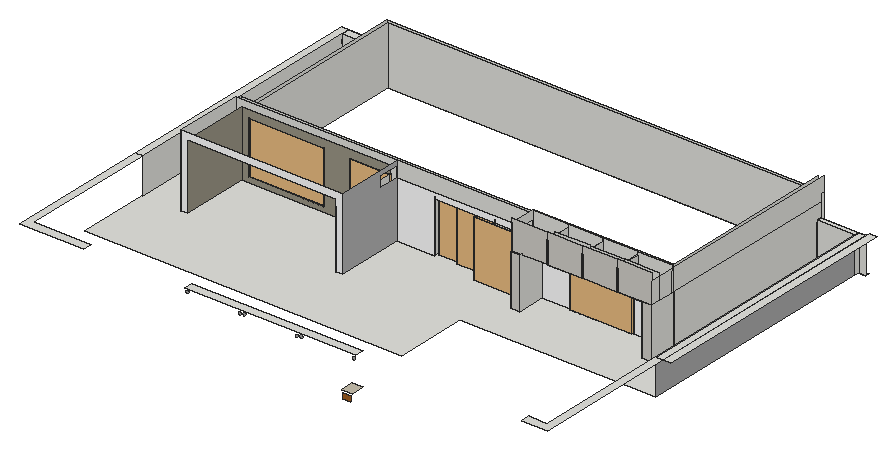
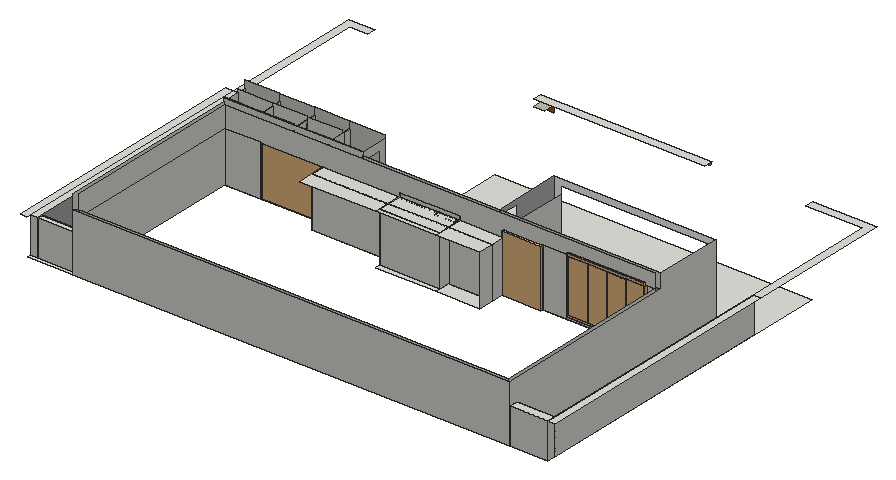
# SketchUp Ruby script. Lengths in inches.
U = 1.inch
M = Sketchup.active_model
def pt(a) = Geom::Point3d.new(a.map { |v| v * U })
def face(e, loops, mat)
  f = e.add_face(loops[0].map { |a| pt(a) })
  loops[1..].each { |l| e.add_face(l.map { |a| pt(a) }).erase! }
  f.material = f.back_material = mat if mat
  f
end
# faces: each face lists its corners as indices into pts; further lists are holes
def faces(e, pts, list, mat = nil) = list.each { |f| face(e, (f[0].is_a?(Array) ? f : [f]).map { |l| l.map { |i| pts[i] } }, mat) }
# xy, xz, yz: faces in a plane at the given z, y or x. An outline is a flat list of corners, or four numbers for a rectangle; further outlines are holes
def ring(l) = l.size == 4 ? [[l[0], l[1]], [l[2], l[1]], [l[2], l[3]], [l[0], l[3]]] : l.each_slice(2).to_a
def flat(e, list, mat, &to3) = list.each { |f| face(e, (f[0].is_a?(Array) ? f : [f]).map { |l| ring(l).map { |u, v| to3.(u, v) } }, mat) }
def xy(e, z, list, mat = nil) = flat(e, list, mat) { |x, y| [x, y, z] }
def xz(e, y, list, mat = nil) = flat(e, list, mat) { |x, z| [x, y, z] }
def yz(e, x, list, mat = nil) = flat(e, list, mat) { |y, z| [x, y, z] }
def lines(e, pts, list) = list.each { |a, b| e.add_line(pt(pts[a]), pt(pts[b])) }
# prism: a flat outline (further loops are holes) pulled along v
def prism(e, loops, v, mat = nil)
  f = face(e, loops, mat); d = Geom::Vector3d.new(v.map { |x| x * U })
  f.pushpull(f.normal.samedirection?(d) ? d.length : -d.length)
end
def box(e, o, s, mat = nil) = prism(e, [[o, [o[0] + s[0], o[1], o[2]], [o[0] + s[0], o[1] + s[1], o[2]], [o[0], o[1] + s[1], o[2]]]], [0, 0, s[2]], mat)
def at(x, y, z, deg = 0) = Geom::Transformation.translation(pt([x, y, z])) * Geom::Transformation.rotation(ORIGIN, Z_AXIS, deg.degrees)
def axes(o, x, y, z) = Geom::Transformation.new([*x, 0, *y, 0, *z, 0, *pt(o).to_a, 1])
def part(name) = M.definitions.add(name)
# library, detail: a bought-in or finely detailed component or shape, given as its bounding box
def library(name, o, s) = part(name).tap { |d| box(d.entities, o, s) }
def detail(e, o, s) = box(e.add_group.entities, o, s)
def put(e, d, t, mat = nil) = e.add_instance(d, t).tap { |i| i.material = mat if mat }
def group(e, t, mat = nil) = e.add_group.tap { |g| g.transformation = t; g.material = mat if mat }.entities
root = M.entities
M.materials.add("Material~3").color = [123, 113, 102]
M.materials.add("[0128_White]").color = [255, 255, 255]
M.materials.add("[0129_WhiteSmoke]").color = [178, 178, 178]
M.materials.add("[0132_LightGray]").color = [169, 169, 169]
M.materials.add("[Concrete Tile]").color = [155, 150, 134]
M.materials.add("[Terrazzo Tile Light]").color = [209, 207, 200]
M.materials.add("[Tile Canvas]").color = [199, 192, 173]
M.materials.add("[Wood Square Tile 02]").color = [160, 95, 34]
c1 = library("3DGeom~4_Defintion",[362.52,-15.59,12.6],[288.85,70.11,1000])
c2 = library("3 door",[0,0,0],[74.8,3.9375,43.31])
c3 = library("door (1)",[38.93,25.48,0],[40,9.94,82.68])
c4 = library("JALI+PATTERN-03",[8.875,53.125,6.4375],[84,1,53.5])
xy(root,5.1875,[[[288.55,611.53,816.46,611.53,816.46,732.28,1144.18,732.28,1144.18,1146.63,1080.92,1146.63,1080.92,851.0625,911.51,851.0625,911.51,845.35,864.05,845.35,864.05,798.41,848.72,798.41,848.72,845.35,784.44,845.35,784.44,874.25,684.16,874.25,684.16,845.35,621.47,845.35,621.47,732.28,610.53,732.28,610.53,851.0625,545.16,851.0625,545.16,845.35,363.11,845.35,363.11,732.28,352.17,732.28,352.17,1146.63,288.55,1146.63],[1065.59,801.78,1080.92,845.35]],[352.17,732.28,352.17,1160.85,1156.17,1160.85,1156.17,1155.13,357.89,1155.13,357.89,851.0625,545.16,851.0625,545.16,845.35,363.11,845.35,363.11,732.28],[610.53,732.28,610.53,846.1,684.16,846.1,684.16,845.35,621.47,845.35,621.47,732.28],[848.72,798.41,848.72,845.35,784.44,845.35,784.44,846.1,911.51,846.1,911.51,845.35,864.05,845.35,864.05,798.41],[1065.59,801.78,1080.92,845.35],
  [610.53,846.1,684.16,874.25],[784.44,846.1,911.51,874.25],[1075.21,851.0625,1080.92,1155.13],[610.53,874.25,684.16,900.375],[684.16,874.25,784.44,892.35],
  [684.16,892.35,784.44,900.375],[288.55,1146.63,352.17,1160.85],[1080.92,1146.63,1144.18,1155.13]])
xy(root,13.84,[[374.83,845.35,499.71,851.0625]])
xy(root,32.74,[[842.6875,453.42,861.125,475.99]],"[Tile Canvas]")
xy(root,65.1875,[[276.92,491.47,382.82,491.47,382.82,505.1,288.55,505.1,288.55,732.28,276.92,732.28],[551.82,491.47,836.67,505.1],[1113.48,491.47,1156.17,491.47,1156.17,732.28,1144.18,732.28,1144.18,505.1,1113.48,505.1],[276.92,732.28,288.55,1160.85],[1144.18,732.28,1156.17,1155.13],
  [1156.87,732.28,1168.49,1160.85],[288.55,1146.63,352.17,1160.85],[1080.92,1146.63,1144.18,1155.13]])
xy(root,89.42,[[848.72,798.41,864.05,801.78],[864.05,801.78,906.77,814.22],[907.71,801.78,911.51,817.6],[911.51,801.78,964.82,817.6],[965.89,801.78,1016.125,817.6],
  [1016.125,801.78,1022.875,817.6],[1024.1875,801.78,1065.59,817.6],[1065.59,801.78,1080.92,817.6],[864.05,814.22,906.77,844.47],[907.71,817.6,911.51,844.47],
  [911.51,817.6,964.82,844.47],[965.89,817.6,1016.125,844.47],[1016.125,817.6,1022.875,844.47],[1024.1875,817.6,1065.59,844.47],[1065.59,817.6,1080.92,844.47],
  [848.72,844.47,864.05,845.35],[864.05,844.47,911.51,845.35],[911.51,844.47,1016.125,845.35],[1016.125,844.47,1065.59,845.35],[1065.59,844.47,1080.92,845.35],
  [684.16,845.35,784.44,846.1],[784.44,845.35,848.72,846.1],[848.72,845.35,911.51,846.1],[911.51,845.35,1016.125,846.1],[1016.125,845.35,1080.92,846.1],
  [610.53,846.1,684.16,851.0625],[784.44,846.1,911.51,851.0625],[911.51,846.1,1016.125,851.0625],[1016.125,846.1,1080.92,851.0625],[610.53,851.0625,684.16,874.25],
  [684.16,851.0625,784.44,874.25],[784.44,851.0625,911.51,874.25],[1075.21,851.0625,1080.92,1155.13],[610.53,874.25,684.16,900.375],[684.16,874.25,784.44,892.35],
  [784.44,874.25,911.51,900.375],[684.16,892.35,784.44,900.375]])
xz(root,453.42,[[845.04,19.53,859.16,29.34]],"[Wood Square Tile 02]")
xz(root,491.47,[[643.03,57.74,643.52,57.8,643.97,57.99,644.36,58.29,644.66,58.68,644.85,59.13,644.91,59.61,644.85,60.1,644.66,60.55,644.36,60.94,643.97,61.24,643.52,61.43,643.03,61.49,642.55,61.43,642.1,61.24,641.71,60.94,641.41,60.55,641.22,60.1,641.16,59.61,641.22,59.13,641.41,58.68,641.71,58.29,642.1,57.99,642.55,57.8],[737.99,57.74,738.47,57.8,738.92,57.99,739.3125,58.29,739.61,58.68,739.8,59.13,739.86,59.61,739.8,60.1,739.61,60.55,739.3125,60.94,738.92,61.24,738.47,61.43,737.99,61.49,737.5,61.43,737.05,61.24,736.66,60.94,736.36,60.55,736.17,60.1,736.11,59.61,736.17,59.13,736.36,58.68,736.66,58.29,737.05,57.99,737.5,57.8],[832.9375,57.74,833.42,57.8,833.875,57.99,834.26,58.29,834.56,58.68,834.75,59.13,834.8125,59.61,834.75,60.1,834.56,60.55,834.26,60.94,833.875,61.24,833.42,61.43,832.9375,61.49,832.45,61.43,832,61.24,831.61,60.94,831.3125,60.55,831.125,60.1,831.0625,59.61,831.125,59.13,831.3125,58.68,831.61,58.29,832,57.99,832.45,57.8],[555.3,59.21,555.79,59.22,556.26,59.36,556.68,59.61,557.02,59.97,557.25,60.4,557.37,60.875,557.35,61.36,557.22,61.83,556.96,62.25,556.61,62.59,556.18,62.82,555.7,62.9375,555.21,62.93,554.74,62.79,554.32,62.53,553.99,62.18,553.75,61.75,553.64,61.27,553.65,60.78,553.79,60.32,554.04,59.9,554.4,59.56,554.83,59.33],[650.25,59.21,650.74,59.22,651.21,59.36,651.63,59.61,651.97,59.97,652.2,60.4,652.32,60.875,652.3,61.36,652.17,61.83,651.91,62.25,651.56,62.59,651.13,62.82,650.65,62.9375,650.16,62.93,649.69,62.79,649.27,62.53,648.9375,62.18,648.7,61.75,648.59,61.27,648.6,60.78,648.74,60.32,648.99,59.9,649.35,59.56,649.78,59.33],
  [745.2,59.21,745.69,59.22,746.16,59.36,746.58,59.61,746.92,59.97,747.15,60.4,747.27,60.875,747.26,61.36,747.12,61.83,746.86,62.25,746.51,62.59,746.08,62.82,745.6,62.9375,745.11,62.93,744.64,62.79,744.23,62.53,743.89,62.18,743.65,61.75,743.54,61.27,743.55,60.78,743.6875,60.32,743.94,59.9,744.3,59.56,744.73,59.33]],"[0132_LightGray]")
xz(root,732.28,[[352.17,5.1875,363.11,5.1875,363.11,114.25,610.53,114.25,610.53,5.1875,621.47,5.1875,621.47,125.1875,352.17,125.1875]],"[0128_White]")
xz(root,798.41,[[848.72,5.1875,864.05,89.42]],"[Terrazzo Tile Light]")
xz(root,801.78,[[1065.59,5.1875,1080.92,89.42],[[848.72,89.42,906.77,138.0625],[852.61,131.88,852.32,131.92,852.05,132.03,851.8125,132.21,851.63,132.44,851.52,132.71,851.48,133,851.52,133.29,851.63,133.57,851.8125,133.8,852.05,133.98,852.32,134.09,852.61,134.13,852.9,134.09,853.17,133.98,853.4,133.8,853.58,133.57,853.69,133.29,853.73,133,853.69,132.71,853.58,132.44,853.4,132.21,853.17,132.03,852.9,131.92],[903.73,131.88,903.44,131.92,903.17,132.03,902.9375,132.21,902.76,132.44,902.65,132.71,902.61,133,902.65,133.29,902.76,133.57,902.9375,133.8,903.17,133.98,903.44,134.09,903.73,134.13,904.02,134.09,904.3,133.98,904.53,133.8,904.71,133.57,904.82,133.29,904.86,133,904.82,132.71,904.71,132.44,904.53,132.21,904.3,132.03,904.02,131.92],[903.73,91.63,903.44,91.67,903.17,91.78,902.9375,91.96,902.76,92.19,902.65,92.46,902.61,92.75,902.65,93.04,902.76,93.32,902.9375,93.55,903.17,93.73,903.44,93.84,903.73,93.88,904.02,93.84,904.3,93.73,904.53,93.55,904.71,93.32,904.82,93.04,904.86,92.75,904.82,92.46,904.71,92.19,904.53,91.96,904.3,91.78,904.02,91.67],[851.55,91.63,851.25,91.67,850.98,91.78,850.75,91.96,850.57,92.19,850.46,92.46,850.42,92.75,850.46,93.04,850.57,93.32,850.75,93.55,850.98,93.73,851.25,93.84,851.55,93.88,851.84,93.84,852.11,93.73,852.34,93.55,852.52,93.32,852.63,93.04,852.67,92.75,852.63,92.46,852.52,92.19,852.34,91.96,852.11,91.78,851.84,91.67]],[[907.71,89.42,964.82,138.0625],[911.6,131.88,911.3,131.92,911.03,132.03,910.8,132.21,910.62,132.44,910.51,132.71,910.47,133,910.51,133.29,910.62,133.57,910.8,133.8,911.03,133.98,911.3,134.09,911.6,134.13,911.89,134.09,912.16,133.98,912.39,133.8,912.57,133.57,912.68,133.29,912.72,133,912.68,132.71,912.57,132.44,912.39,132.21,912.16,132.03,911.89,131.92],[962.72,91.63,962.43,91.67,962.16,91.78,961.93,91.96,961.75,92.19,961.63,92.46,961.6,92.75,961.63,93.04,961.75,93.32,961.93,93.55,962.16,93.73,962.43,93.84,962.72,93.88,963.01,93.84,963.28,93.73,963.52,93.55,963.7,93.32,963.81,93.04,963.85,92.75,963.81,92.46,963.7,92.19,963.52,91.96,963.28,91.78,963.01,91.67],[910.53,91.63,910.24,91.67,909.97,91.78,909.74,91.96,909.56,92.19,909.45,92.46,909.41,92.75,909.45,93.04,909.56,93.32,909.74,93.55,909.97,93.73,910.24,93.84,910.53,93.88,910.82,93.84,911.1,93.73,911.33,93.55,911.51,93.32,911.62,93.04,911.66,92.75,911.62,92.46,911.51,92.19,911.33,91.96,911.1,91.78,910.82,91.67],[962.72,131.88,962.43,131.92,962.16,132.03,961.93,132.21,961.75,132.44,961.63,132.71,961.6,133,961.63,133.29,961.75,133.57,961.93,133.8,962.16,133.98,962.43,134.09,962.72,134.13,963.01,134.09,963.28,133.98,963.52,133.8,963.7,133.57,963.81,133.29,963.85,133,963.81,132.71,963.7,132.44,963.52,132.21,963.28,132.03,963.01,131.92]],[[965.89,89.42,1022.875,138.0625],[1020.9,131.88,1020.61,131.92,1020.33,132.03,1020.1,132.21,1019.92,132.44,1019.81,132.71,1019.77,133,1019.81,133.29,1019.92,133.57,1020.1,133.8,1020.33,133.98,1020.61,134.09,1020.9,134.13,1021.1875,134.09,1021.46,133.98,1021.69,133.8,1021.87,133.57,1021.98,133.29,1022.02,133,1021.98,132.71,1021.87,132.44,1021.69,132.21,1021.46,132.03,1021.1875,131.92],[969.77,131.88,969.48,131.92,969.21,132.03,968.98,132.21,968.8,132.44,968.69,132.71,968.65,133,968.69,133.29,968.8,133.57,968.98,133.8,969.21,133.98,969.48,134.09,969.77,134.13,970.0625,134.09,970.33,133.98,970.57,133.8,970.75,133.57,970.86,133.29,970.9,133,970.86,132.71,970.75,132.44,970.57,132.21,970.33,132.03,970.0625,131.92],[1020.9,91.63,1020.61,91.67,1020.33,91.78,1020.1,91.96,1019.92,92.19,1019.81,92.46,1019.77,92.75,1019.81,93.04,1019.92,93.32,1020.1,93.55,1020.33,93.73,1020.61,93.84,1020.9,93.88,1021.1875,93.84,1021.46,93.73,1021.69,93.55,1021.87,93.32,1021.98,93.04,1022.02,92.75,1021.98,92.46,1021.87,92.19,1021.69,91.96,1021.46,91.78,1021.1875,91.67],[968.71,91.63,968.42,91.67,968.15,91.78,967.91,91.96,967.74,92.19,967.62,92.46,967.58,92.75,967.62,93.04,967.74,93.32,967.91,93.55,968.15,93.73,968.42,93.84,968.71,93.88,969,93.84,969.27,93.73,969.5,93.55,969.68,93.32,969.8,93.04,969.83,92.75,969.8,92.46,969.68,92.19,969.5,91.96,969.27,91.78,969,91.67]],[[1024.1875,89.42,1080.92,138.0625],[1027.01,91.63,1026.72,91.67,1026.45,91.78,1026.21,91.96,1026.04,92.19,1025.92,92.46,1025.89,92.75,1025.92,93.04,1026.04,93.32,1026.21,93.55,1026.45,93.73,1026.72,93.84,1027.01,93.88,1027.3,93.84,1027.57,93.73,1027.81,93.55,1027.98,93.32,1028.1,93.04,1028.14,92.75,1028.1,92.46,1027.98,92.19,1027.81,91.96,1027.57,91.78,1027.3,91.67],[1028.07,131.88,1027.78,131.92,1027.51,132.03,1027.28,132.21,1027.1,132.44,1026.99,132.71,1026.95,133,1026.99,133.29,1027.1,133.57,1027.28,133.8,1027.51,133.98,1027.78,134.09,1028.07,134.13,1028.36,134.09,1028.64,133.98,1028.87,133.8,1029.05,133.57,1029.16,133.29,1029.2,133,1029.16,132.71,1029.05,132.44,1028.87,132.21,1028.64,132.03,1028.36,131.92],[1079.2,91.63,1078.91,91.67,1078.64,91.78,1078.4,91.96,1078.22,92.19,1078.11,92.46,1078.07,92.75,1078.11,93.04,1078.22,93.32,1078.4,93.55,1078.64,93.73,1078.91,93.84,1079.2,93.88,1079.49,93.84,1079.76,93.73,1079.99,93.55,1080.17,93.32,1080.28,93.04,1080.32,92.75,1080.28,92.46,1080.17,92.19,1079.99,91.96,1079.76,91.78,1079.49,91.67],[1079.2,131.88,1078.91,131.92,1078.64,132.03,1078.4,132.21,1078.22,132.44,1078.11,132.71,1078.07,133,1078.11,133.29,1078.22,133.57,1078.4,133.8,1078.64,133.98,1078.91,134.09,1079.2,134.13,1079.49,134.09,1079.76,133.98,1079.99,133.8,1080.17,133.57,1080.28,133.29,1080.32,133,1080.28,132.71,1080.17,132.44,1079.99,132.21,1079.76,132.03,1079.49,131.92]]],"[Terrazzo Tile Light]")
xz(root,817.6,[[907.71,89.42,964.82,131.1875],[965.89,89.42,1022.875,131.1875],[1024.1875,89.42,1080.92,131.1875]])
xz(root,844.47,[[848.72,89.42,906.77,131.1875],[906.77,89.42,907.71,131.1875],[907.71,89.42,964.82,131.1875],[964.82,89.42,965.89,131.1875],[965.89,89.42,1022.875,131.1875],
  [1022.875,89.42,1024.1875,131.1875],[1024.1875,89.42,1080.92,131.1875]])
xz(root,845.35,[[784.44,5.1875,848.72,89.42],[1065.59,5.1875,1080.92,89.42]])
xz(root,845.35,[[621.47,5.1875,684.16,5.1875,684.16,89.42,848.72,89.42,848.72,99.26,621.47,99.26],[864.05,5.1875,911.51,89.42],[1016.125,5.1875,1065.59,89.42]],"[0128_White]")
xz(root,845.35,[[[363.11,5.1875,545.16,5.1875,545.16,101.375,610.53,101.375,610.53,114.25,363.11,114.25],[374.83,13.84,499.71,101.78]]],"[Concrete Tile]")
xz(root,846.1,[[610.53,5.1875,684.16,89.42],[784.44,5.1875,911.51,89.42],[610.53,89.42,621.47,89.42,621.47,125.1875,352.17,125.1875,352.17,101.375,610.53,101.375],[621.47,89.42,621.47,125.1875,848.72,125.1875,848.72,89.42,784.44,89.42,784.44,95.79,684.16,95.79,684.16,89.42],[684.16,89.42,784.44,95.79],
  [848.72,89.42,1080.92,131.1875]])
xz(root,851.0625,[[357.89,5.1875,357.89,101.375,374.83,101.375,374.83,13.84,499.71,13.84,499.71,101.375,545.16,101.375,545.16,5.1875],[1016.125,5.1875,1075.21,89.42],[1075.21,5.1875,1080.92,89.42],[610.53,89.42,610.53,101.375,499.71,101.375,499.71,101.78,374.83,101.78,374.83,101.375,357.89,101.375,357.89,125.1875,1075.21,125.1875,1075.21,89.42,784.44,89.42,784.44,95.79,684.16,95.79,684.16,89.42],[684.16,89.42,784.44,95.79]])
xz(root,874.25,[[610.53,5.1875,911.51,89.42]])
xz(root,892.35,[[684.16,5.1875,784.44,89.42]])
xz(root,1146.63,[[288.55,5.1875,352.17,65.1875],[1080.92,5.1875,1144.18,65.1875]])
xz(root,1155.13,[[357.89,5.1875,1075.21,101.375],[1075.21,5.1875,1080.92,89.42],[1080.92,5.1875,1144.18,65.1875],[1144.18,5.1875,1156.17,65.1875],[1075.21,89.42,1080.92,101.375]])
xz(root,1160.85,[[288.55,5.1875,352.17,65.1875],[352.17,5.1875,1080.92,101.375]])
yz(root,288.55,[[732.28,5.1875,1146.63,65.1875],[1146.63,5.1875,1160.85,65.1875]])
yz(root,352.17,[[732.28,5.1875,732.28,125.1875,846.1,125.1875,846.1,101.375,1160.85,101.375,1160.85,65.1875,1146.63,65.1875,1146.63,5.1875],[1146.63,5.1875,1160.85,65.1875]])
yz(root,357.89,[[851.0625,5.1875,1155.13,101.375]])
yz(root,363.11,[[732.28,5.1875,845.35,114.25]],"[Concrete Tile]")
yz(root,374.83,[[845.35,13.84,851.0625,101.78]])
yz(root,499.71,[[845.35,13.84,851.0625,101.78]])
yz(root,545.16,[[845.35,5.1875,851.0625,101.375]])
yz(root,610.53,[[732.28,5.1875,846.1,101.375],[846.1,5.1875,874.25,89.42],[874.25,5.1875,900.375,89.42],[846.1,89.42,851.0625,101.375]])
yz(root,621.47,[[845.35,89.42,846.1,125.1875]])
yz(root,621.47,[[732.28,5.1875,845.35,5.1875,845.35,99.26,810.97,99.26,810.97,117.26,845.35,117.26,845.35,125.1875,732.28,125.1875]],"[0129_WhiteSmoke]")
yz(root,684.16,[[845.35,5.1875,846.1,89.42],[846.1,5.1875,892.35,89.42],[846.1,89.42,851.0625,95.79]])
yz(root,784.44,[[845.35,5.1875,846.1,89.42],[846.1,5.1875,892.35,89.42],[846.1,89.42,851.0625,95.79]])
yz(root,848.72,[[798.41,5.1875,798.41,89.42,801.78,89.42,801.78,131.1875,844.47,131.1875,844.47,117.26,810.97,117.26,810.97,99.26,844.47,99.26,844.47,89.42,845.35,89.42,845.35,5.1875],[844.47,89.42,845.35,99.26],[845.35,89.42,846.1,125.1875]])
yz(root,864.05,[[798.41,5.1875,845.35,89.42]])
yz(root,906.77,[[801.78,89.42,814.22,125.1875],[814.22,89.42,844.47,125.1875]])
yz(root,907.71,[[801.78,89.42,817.6,125.1875],[817.6,89.42,844.47,125.1875]])
yz(root,911.51,[[845.35,5.1875,846.1,89.42],[846.1,5.1875,874.25,89.42]])
yz(root,964.82,[[801.78,89.42,817.6,125.1875],[817.6,89.42,844.47,125.1875]])
yz(root,965.89,[[801.78,89.42,817.6,125.1875],[817.6,89.42,844.47,125.1875]])
yz(root,1016.125,[[845.35,5.1875,851.0625,89.42]])
yz(root,1022.875,[[801.78,89.42,817.6,125.1875],[817.6,89.42,844.47,125.1875]])
yz(root,1024.1875,[[801.78,89.42,817.6,125.1875],[817.6,89.42,844.47,125.1875]])
yz(root,1065.59,[[801.78,5.1875,845.35,89.42]])
yz(root,1075.21,[[851.0625,5.1875,1155.13,89.42],[851.0625,89.42,1155.13,125.1875]])
yz(root,1080.92,[[801.78,5.1875,845.35,89.42],[851.0625,5.1875,1146.63,5.1875,1146.63,65.1875,1155.13,65.1875,1155.13,89.42,851.0625,89.42],[1146.63,5.1875,1155.13,65.1875],[801.78,89.42,817.6,125.1875],[817.6,89.42,844.47,125.1875],
  [844.47,89.42,846.1,125.1875],[846.1,89.42,1155.13,89.42,1155.13,101.375,1160.85,101.375,1160.85,125.1875,846.1,125.1875]])
yz(root,1144.18,[[1146.63,5.1875,1155.13,65.1875]])
yz(root,1144.18,[[732.28,5.1875,1146.63,65.1875]],"[0132_LightGray]")
p = [[848.72,814.22,89.42],[864.05,814.22,89.42]]
lines(root,p,[[0,1]])
put(root,c1,axes([332.23,853.3125,12.94],[0.11056,0,0],[0,-0.05859,0],[0,0,0.08734]),"Material~3")
put(root,c1,axes([363.7,853.99,12.94],[0.11056,0,0],[0,-0.05859,0],[0,0,0.08734]),"Material~3")
put(root,c2,axes([374.83,847.72,10.15],[1.71563,0,0],[0,1.38,0],[0,0,2.21476]))
put(root,c1,axes([395.76,853.99,12.94],[0.11056,0,0],[0,-0.05859,0],[0,0,0.08734]),"Material~3")
put(root,c1,axes([427.83,853.99,12.94],[0.11056,0,0],[0,-0.05859,0],[0,0,0.08734]),"Material~3")
put(root,c3,axes([481.54,814.19,5.1875],[1.63437,0,0],[0,1.16,0],[0,0,1.16]))
put(root,c1,axes([647.11,857.09,3.96],[0.11056,0,0],[0,-0.11056,0],[0,0,0.08439]),"Material~3")
put(root,c1,axes([680.49,851.7,3.96],[0.11056,0,0],[0,-0.08955,0],[0,0,0.08439]),"Material~3")
put(root,c1,axes([712.43,851.7,3.96],[0.11056,0,0],[0,-0.08955,0],[0,0,0.08439]),"Material~3")
put(root,c4,axes([754.07,766.91,109.2],[0,0,-1.12],[0,1.12,0],[1.5792,0,0]))
put(root,c2,axes([911.51,843.85,5.1875],[1.38,0,0],[0,1.38,0],[0,0,1.94496]))
